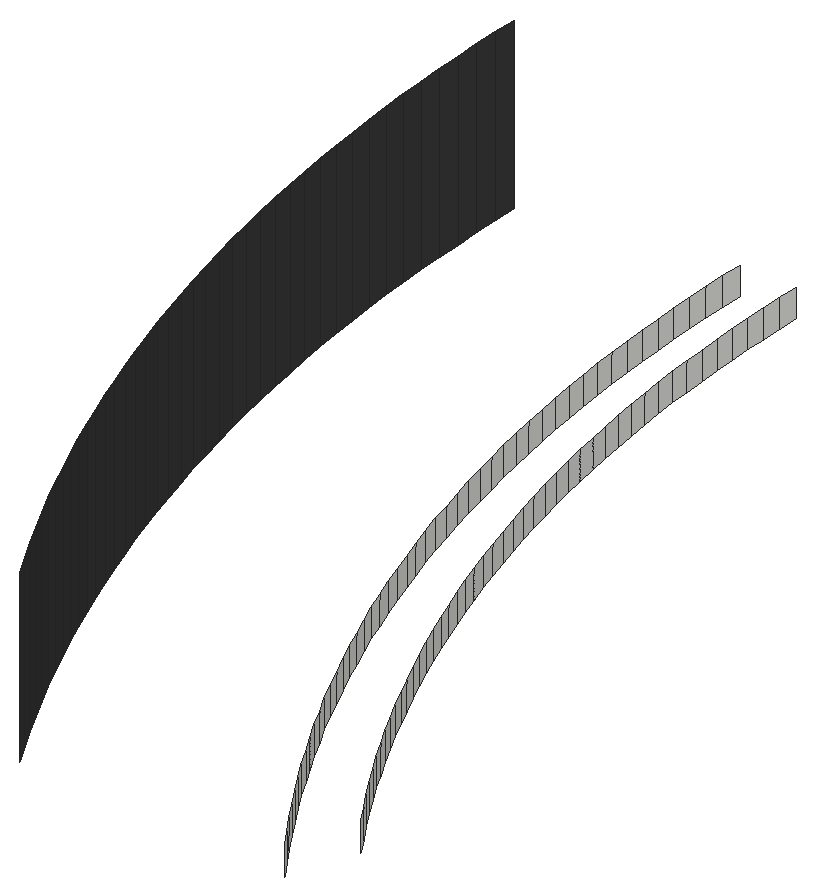
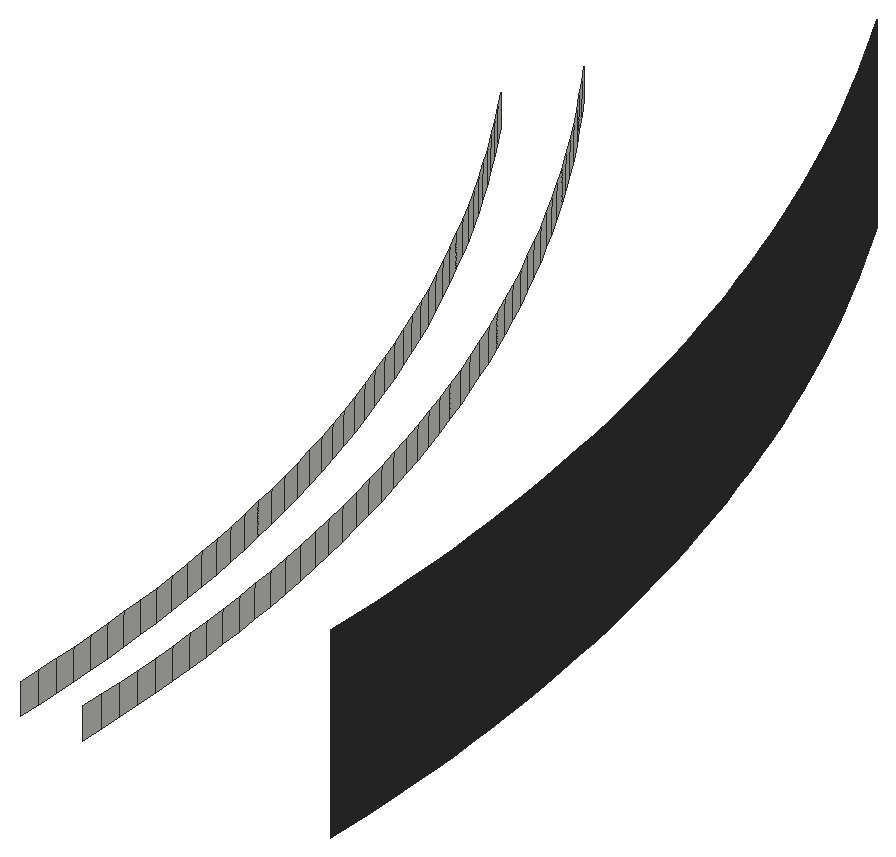
# SketchUp Ruby script. Lengths in inches.
U = 1.inch
M = Sketchup.active_model
def pt(a) = Geom::Point3d.new(a.map { |v| v * U })
def face(e, loops, mat)
  f = e.add_face(loops[0].map { |a| pt(a) })
  loops[1..].each { |l| e.add_face(l.map { |a| pt(a) }).erase! }
  f.material = f.back_material = mat if mat
  f
end
# faces: each face lists its corners as indices into pts; further lists are holes
def faces(e, pts, list, mat = nil) = list.each { |f| face(e, (f[0].is_a?(Array) ? f : [f]).map { |l| l.map { |i| pts[i] } }, mat) }
# xy, xz, yz: faces in a plane at the given z, y or x. An outline is a flat list of corners, or four numbers for a rectangle; further outlines are holes
def ring(l) = l.size == 4 ? [[l[0], l[1]], [l[2], l[1]], [l[2], l[3]], [l[0], l[3]]] : l.each_slice(2).to_a
def flat(e, list, mat, &to3) = list.each { |f| face(e, (f[0].is_a?(Array) ? f : [f]).map { |l| ring(l).map { |u, v| to3.(u, v) } }, mat) }
def xy(e, z, list, mat = nil) = flat(e, list, mat) { |x, y| [x, y, z] }
def xz(e, y, list, mat = nil) = flat(e, list, mat) { |x, z| [x, y, z] }
def yz(e, x, list, mat = nil) = flat(e, list, mat) { |y, z| [x, y, z] }
def lines(e, pts, list) = list.each { |a, b| e.add_line(pt(pts[a]), pt(pts[b])) }
# prism: a flat outline (further loops are holes) pulled along v
def prism(e, loops, v, mat = nil)
  f = face(e, loops, mat); d = Geom::Vector3d.new(v.map { |x| x * U })
  f.pushpull(f.normal.samedirection?(d) ? d.length : -d.length)
end
def box(e, o, s, mat = nil) = prism(e, [[o, [o[0] + s[0], o[1], o[2]], [o[0] + s[0], o[1] + s[1], o[2]], [o[0], o[1] + s[1], o[2]]]], [0, 0, s[2]], mat)
def at(x, y, z, deg = 0) = Geom::Transformation.translation(pt([x, y, z])) * Geom::Transformation.rotation(ORIGIN, Z_AXIS, deg.degrees)
def axes(o, x, y, z) = Geom::Transformation.new([*x, 0, *y, 0, *z, 0, *pt(o).to_a, 1])
def part(name) = M.definitions.add(name)
# library, detail: a bought-in or finely detailed component or shape, given as its bounding box
def library(name, o, s) = part(name).tap { |d| box(d.entities, o, s) }
def detail(e, o, s) = box(e.add_group.entities, o, s)
def put(e, d, t, mat = nil) = e.add_instance(d, t).tap { |i| i.material = mat if mat }
def group(e, t, mat = nil) = e.add_group.tap { |g| g.transformation = t; g.material = mat if mat }.entities
root = M.entities
M.materials.add("1496 AP 8293 CARBON COPY").color = [58, 58, 58]
yz(root,11,[[96.57,258,97,261]],"1496 AP 8293 CARBON COPY")
yz(root,15,[[96.62,258,97,258.5]])
yz(root,16,[[96.63,258,97,258.5]])
p = [[20.32,80.26,258],[20.1,80.57,258],[20.1,80.57,258.5],[20.32,80.26,258.5],[15.42,80.5,261],[15.21,80.875,261],
  [15.21,80.875,258],[15.42,80.5,258],[19.89,80.89,258],[19.89,80.89,258.5],[15,81.25,261],[15,81.25,258],
  [19.68,81.21,258],[19.68,81.21,258.5],[19.47,81.53,258],[19.47,81.53,258.5],[14.8,81.63,261],[14.8,81.63,258],
  [20.52,81.75,258],[20.72,81.44,258],[20.72,81.44,258.5],[20.52,81.75,258.5],[19.27,81.85,258],[19.27,81.85,258.5],
  [14.6,82.02,261],[14.6,82.02,258],[19.08,82.17,258],[19.08,82.17,258.5],[20.32,82.06,258],[20.32,82.06,258.5],
  [14.4,82.4,261],[14.4,82.4,258],[20.125,82.37,258],[20.125,82.37,258.5],[18.89,82.5,258],[18.89,82.5,258.5],
  [14.21,82.79,261],[14.21,82.79,258],[19.9375,82.68,258],[19.9375,82.68,258.5],[18.7,82.83,258],[18.7,82.83,258.5],
  [19.75,83,258],[19.75,83,258.5],[14.03,83.18,261],[14.03,83.18,258],[18.51,83.16,258],[18.51,83.16,258.5],
  [19.57,83.32,258],[19.57,83.32,258.5],[13.85,83.58,261],[13.85,83.58,258],[18.34,83.5,258],[18.34,83.5,258.5],
  [19.39,83.64,258],[19.39,83.64,258.5],[18.16,83.83,258],[18.16,83.83,258.5],[13.68,83.97,261],[13.68,83.97,258],
  [19.22,83.96,258],[19.22,83.96,258.5],[17.99,84.17,258],[17.99,84.17,258.5],[13.51,84.37,261],[13.51,84.37,258],
  [19.05,84.29,258],[19.05,84.29,258.5],[17.83,84.52,258],[17.83,84.52,258.5],[18.89,84.62,258],[18.89,84.62,258.5],
  [13.35,84.77,261],[13.35,84.77,258],[17.66,84.86,258],[17.66,84.86,258.5],[18.73,84.95,258],[18.73,84.95,258.5],
  [13.19,85.17,261],[13.19,85.17,258],[17.51,85.2,258],[17.51,85.2,258.5],[18.57,85.28,258],[18.57,85.28,258.5],
  [13.04,85.58,261],[13.04,85.58,258],[17.36,85.55,258],[17.36,85.55,258.5],[18.42,85.61,258],[18.42,85.61,258.5],
  [12.89,85.98,261],[12.89,85.98,258],[17.21,85.9,258],[17.21,85.9,258.5],[18.27,85.95,258],[18.27,85.95,258.5],
  [17.06,86.25,258],[17.06,86.25,258.5],[18.13,86.28,258],[18.13,86.28,258.5],[12.75,86.39,261],[12.75,86.39,258],
  [16.93,86.61,258],[16.93,86.61,258.5],[17.99,86.625,258],[17.99,86.625,258.5],[12.62,86.8,261],[12.62,86.8,258],
  [16.79,86.96,258],[16.79,86.96,258.5],[17.86,86.97,258],[17.86,86.97,258.5],[12.48,87.21,261],[12.48,87.21,258],
  [16.66,87.32,258],[16.66,87.32,258.5],[17.73,87.31,258],[17.73,87.31,258.5],[12.36,87.63,261],[12.36,87.63,258],
  [16.54,87.68,258],[16.54,87.68,258.5],[17.61,87.65,258],[17.61,87.65,258.5],[12.24,88.04,261],[12.24,88.04,258],
  [16.42,88.04,258],[16.42,88.04,258.5],[17.49,88,258],[17.49,88,258.5],[12.125,88.46,261],[12.125,88.46,258],
  [16.3,88.4,258],[16.3,88.4,258.5],[17.37,88.35,258],[17.37,88.35,258.5],[17.26,88.7,258],[17.26,88.7,258.5],
  [16.19,88.76,258],[16.19,88.76,258.5],[12.02,88.875,261],[12.02,88.875,258],[17.15,89.05,258],[17.15,89.05,258.5],
  [16.09,89.13,258],[16.09,89.13,258.5],[11.91,89.3,261],[11.91,89.3,258],[17.05,89.4,258],[17.05,89.4,258.5],
  [15.99,89.49,258],[15.99,89.49,258.5],[11.8125,89.72,261],[11.8125,89.72,258],[16.95,89.75,258],[16.95,89.75,258.5],
  [15.89,89.86,258],[15.89,89.86,258.5],[11.72,90.14,261],[11.72,90.14,258],[16.86,90.11,258],[16.86,90.11,258.5],
  [15.8,90.23,258],[15.8,90.23,258.5],[11.63,90.5625,261],[11.63,90.5625,258],[16.77,90.46,258],[16.77,90.46,258.5],
  [15.72,90.6,258],[15.72,90.6,258.5],[16.69,90.82,258],[16.69,90.82,258.5],[11.55,90.99,261],[11.55,90.99,258],
  [15.63,90.97,258],[15.63,90.97,258.5],[16.61,91.18,258],[16.61,91.18,258.5],[11.48,91.41,261],[11.48,91.41,258],
  [15.56,91.34,258],[15.56,91.34,258.5],[16.54,91.54,258],[16.54,91.54,258.5],[15.49,91.72,258],[15.49,91.72,258.5],
  [11.41,91.84,261],[11.41,91.84,258],[16.47,91.9,258],[16.47,91.9,258.5],[15.42,92.09,258],[15.42,92.09,258.5],
  [11.34,92.26,261],[11.34,92.26,258],[16.4,92.26,258],[16.4,92.26,258.5],[15.36,92.46,258],[15.36,92.46,258.5],
  [11.28,92.69,261],[11.28,92.69,258],[16.34,92.62,258],[16.34,92.62,258.5],[15.3,92.84,258],[15.3,92.84,258.5],
  [16.29,92.98,258],[16.29,92.98,258.5],[11.23,93.12,261],[11.23,93.12,258],[15.25,93.21,258],[15.25,93.21,258.5],
  [16.24,93.35,258],[16.24,93.35,258.5],[11.18,93.55,261],[11.18,93.55,258],[15.2,93.59,258],[15.2,93.59,258.5],
  [16.19,93.71,258],[16.19,93.71,258.5],[11.14,93.98,261],[11.14,93.98,258],[15.16,93.97,258],[15.16,93.97,258.5],
  [16.15,94.07,258],[16.15,94.07,258.5],[11.1,94.41,261],[11.1,94.41,258],[15.12,94.35,258],[15.12,94.35,258.5],
  [16.12,94.4375,258],[16.12,94.4375,258.5],[15.09,94.72,258],[15.09,94.72,258.5],[11.07,94.84,261],[11.07,94.84,258],
  [16.09,94.8,258],[16.09,94.8,258.5],[15.0625,95.1,258],[15.0625,95.1,258.5],[11.05,95.27,261],[11.05,95.27,258],
  [16.06,95.17,258],[16.06,95.17,258.5],[15.04,95.48,258],[15.04,95.48,258.5],[16.04,95.53,258],[16.04,95.53,258.5],
  [11.03,95.7,261],[11.03,95.7,258],[15.02,95.86,258],[15.02,95.86,258.5],[16.02,95.9,258],[16.02,95.9,258.5],
  [11.01,96.14,261],[11.01,96.14,258],[15.01,96.24,258],[15.01,96.24,258.5],[16.01,96.27,258],[16.01,96.27,258.5],
  [11,96.57,261],[11,96.57,258],[15,96.62,258],[15,96.62,258.5],[16,96.63,258],[16,96.63,258.5]]
faces(root,p,[[0,1,2,3],[1,8,9,2],[8,12,13,9],[12,14,15,13],[18,19,20,21],[14,22,23,15],[22,26,27,23],[28,18,21,29],
  [32,28,29,33],[26,34,35,27],[38,32,33,39],[34,40,41,35],[42,38,39,43],[40,46,47,41],[48,42,43,49],[46,52,53,47],
  [54,48,49,55],[52,56,57,53],[60,54,55,61],[56,62,63,57],[66,60,61,67],[62,68,69,63],[70,66,67,71],[68,74,75,69],
  [76,70,71,77],[74,80,81,75],[82,76,77,83],[80,86,87,81],[88,82,83,89],[86,92,93,87],[94,88,89,95],[92,96,97,93],
  [98,94,95,99],[96,102,103,97],[104,98,99,105],[102,108,109,103],[110,104,105,111],[108,114,115,109],[116,110,111,117],[114,120,121,115],
  [122,116,117,123],[120,126,127,121],[128,122,123,129],[126,132,133,127],[134,128,129,135],[136,134,135,137],[132,138,139,133],[142,136,137,143],
  [138,144,145,139],[148,142,143,149],[144,150,151,145],[154,148,149,155],[150,156,157,151],[160,154,155,161],[156,162,163,157],[166,160,161,167],
  [162,168,169,163],[170,166,167,171],[168,174,175,169],[176,170,171,177],[174,180,181,175],[182,176,177,183],[180,184,185,181],[188,182,183,189],
  [184,190,191,185],[194,188,189,195],[190,196,197,191],[200,194,195,201],[196,202,203,197],[204,200,201,205],[202,208,209,203],[210,204,205,211],
  [208,214,215,209],[216,210,211,217],[214,220,221,215],[222,216,217,223],[220,226,227,221],[228,222,223,229],[226,230,231,227],[234,228,229,235],
  [230,236,237,231],[240,234,235,241],[236,242,243,237],[244,240,241,245],[242,248,249,243],[250,244,245,251],[248,254,255,249],[256,250,251,257],
  [254,260,261,255],[262,256,257,263]])
faces(root,p,[[4,5,6,7],[5,10,11,6],[10,16,17,11],[16,24,25,17],[24,30,31,25],[30,36,37,31],[36,44,45,37],[44,50,51,45],
  [50,58,59,51],[58,64,65,59],[64,72,73,65],[72,78,79,73],[78,84,85,79],[84,90,91,85],[90,100,101,91],[100,106,107,101],
  [106,112,113,107],[112,118,119,113],[118,124,125,119],[124,130,131,125],[130,140,141,131],[140,146,147,141],[146,152,153,147],[152,158,159,153],
  [158,164,165,159],[164,172,173,165],[172,178,179,173],[178,186,187,179],[186,192,193,187],[192,198,199,193],[198,206,207,199],[206,212,213,207],
  [212,218,219,213],[218,224,225,219],[224,232,233,225],[232,238,239,233],[238,246,247,239],[246,252,253,247],[252,258,259,253]],"1496 AP 8293 CARBON COPY")
